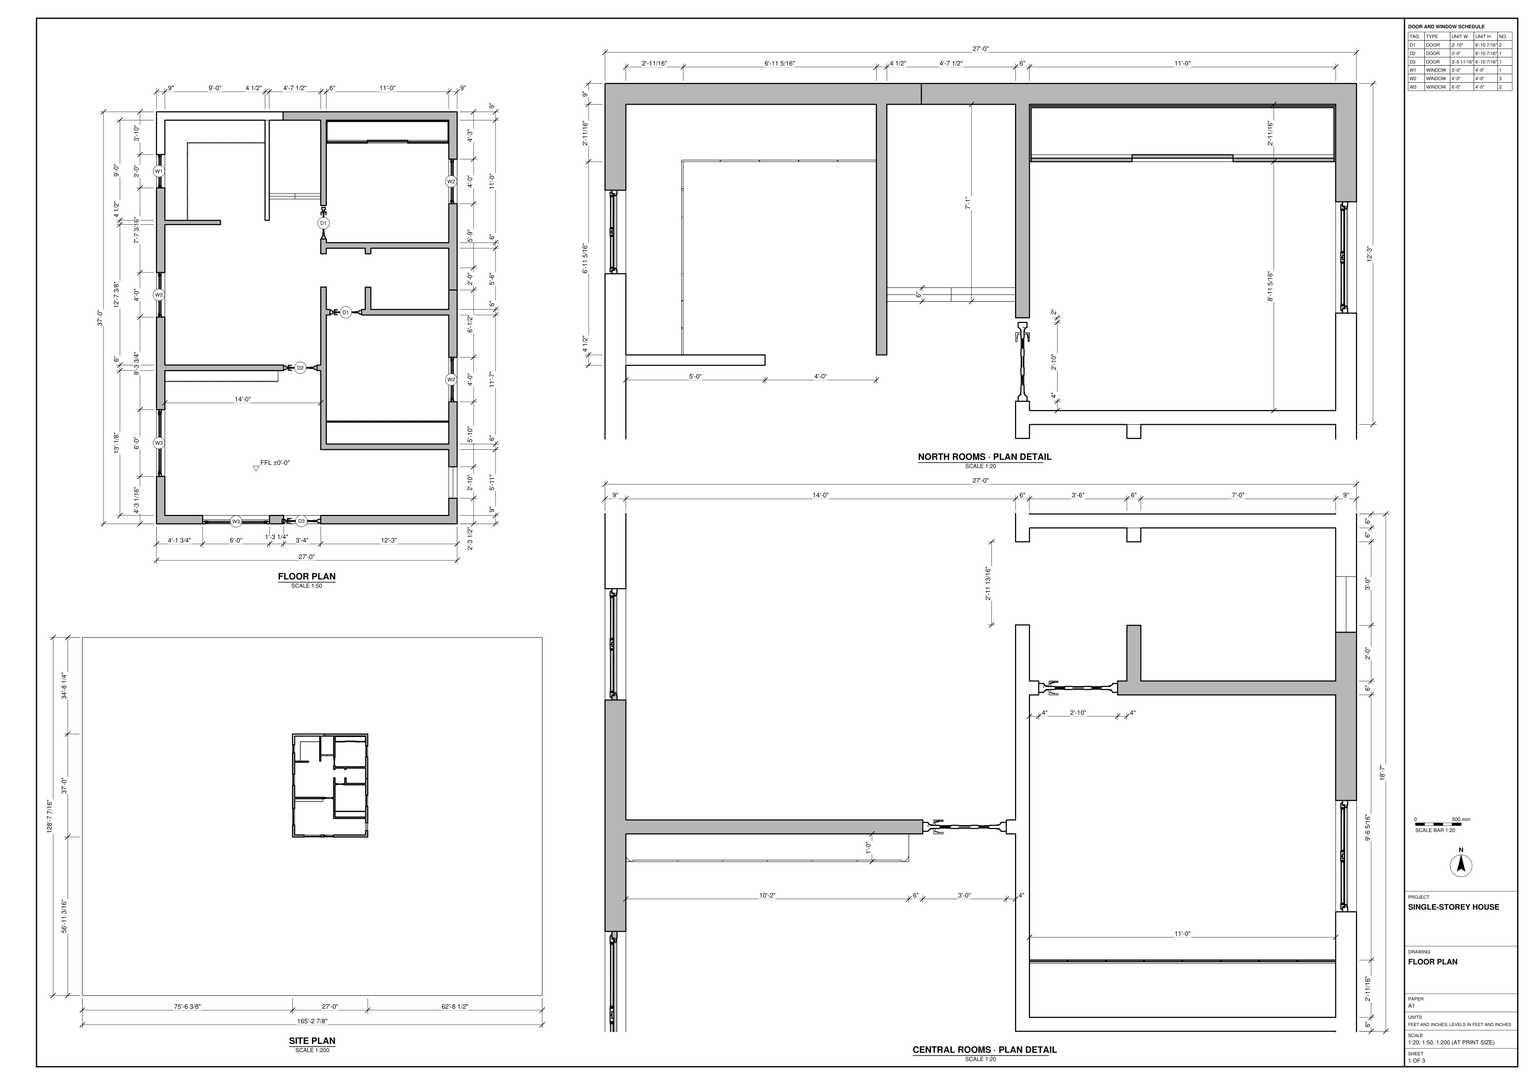
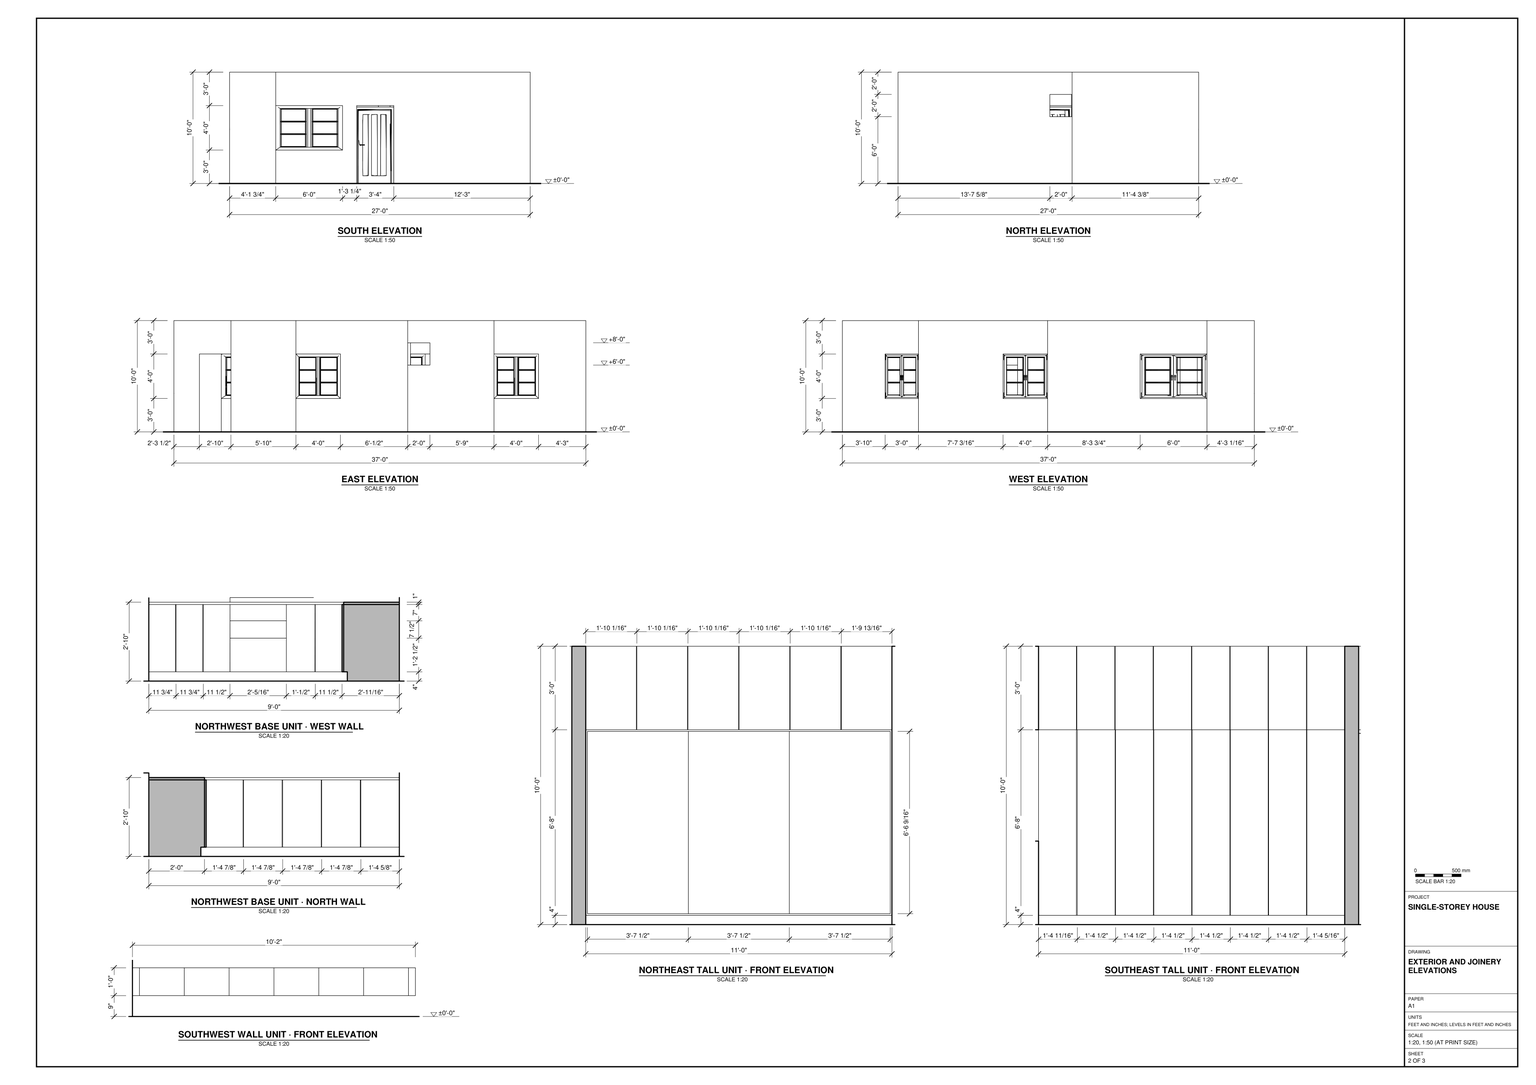
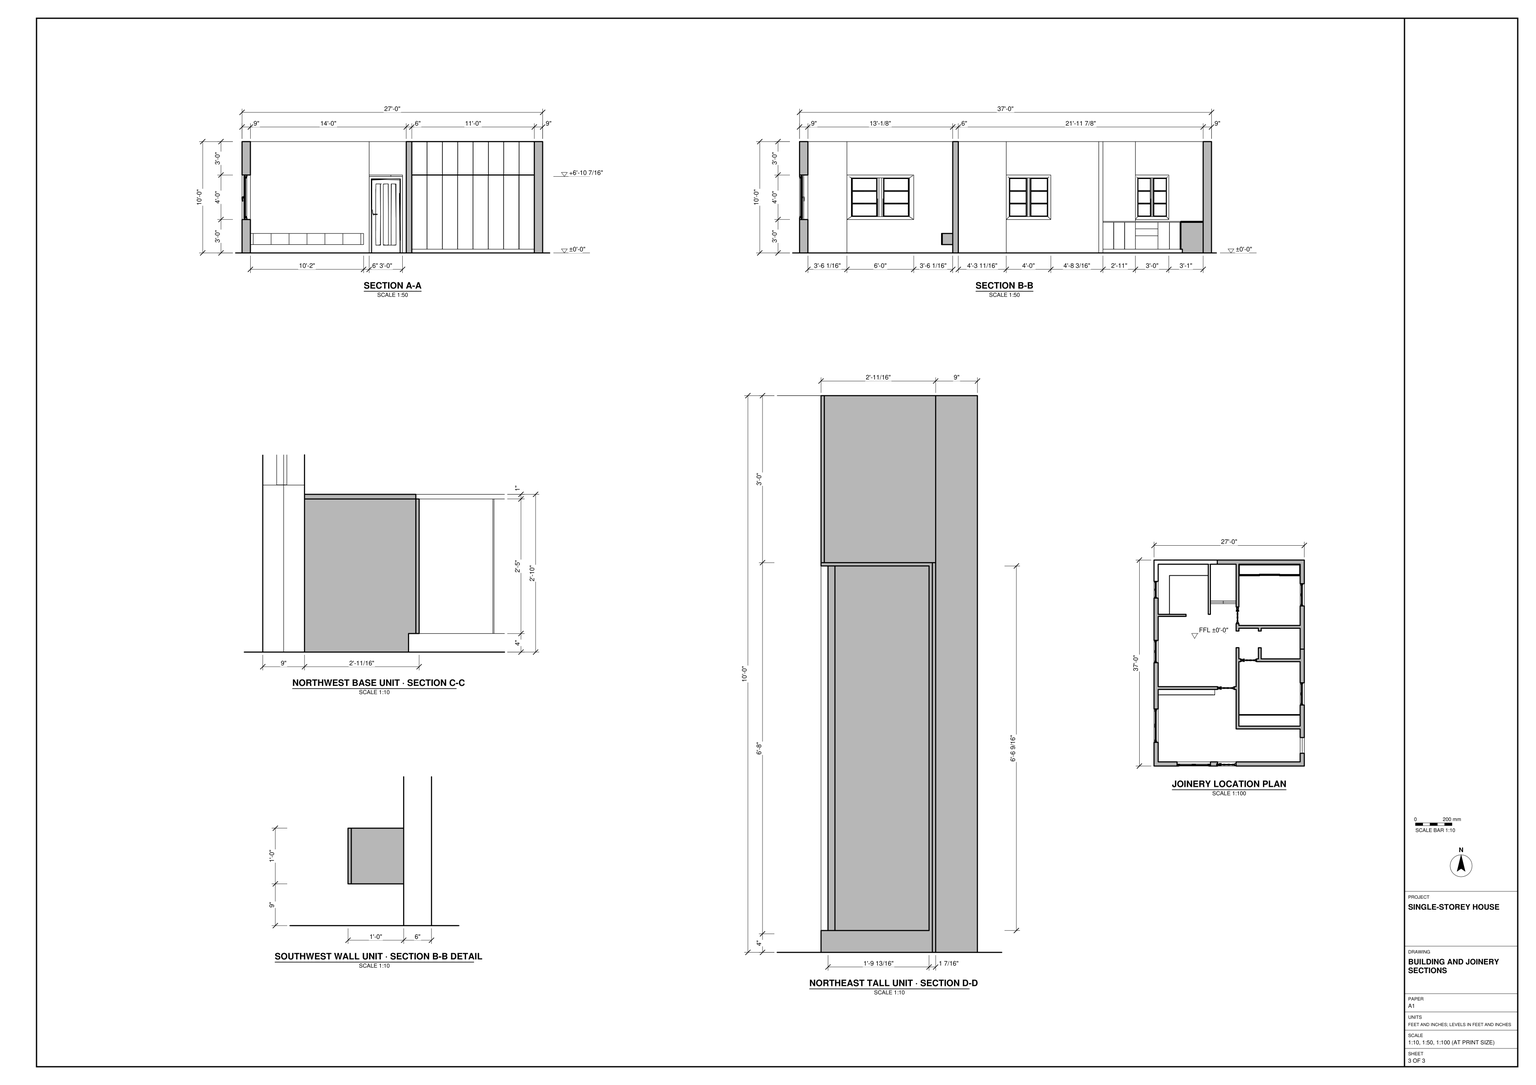
Build the house and its rectangular site in SketchUp from task_files/diagram_01.pdf. Work in feet and inches. The overall model measures 165'-2 7/8" east to west, 128'-7 7/16" north to south and 10'-0" high. The house footprint is 27'-0" east to west by 37'-0" north to south. Use the setbacks on the site plan to position it, with the entrance on the south side and the single finished floor at ±0'-0".

Model the floor, the 9" exterior walls and the interior partitions at their drawn thicknesses. Use the enlarged plans to locate the partition ends, doorways and passages between rooms. Fit the scheduled doors and windows, and use the elevations to set the sill heights and locate the smaller high openings on the north and east walls.

Build the base cabinetry around the northwest corner, the low wall-mounted unit in the southwest room and the full-height storage units in the northeast and southeast rooms. Follow the joinery elevations for the panel divisions and the sections for the cabinet depths, plinths and clearance above the floor. Keep shell elements and individual joinery pieces in separate groups or components, and use components for repeated parts. Decor and loose items, where shown, may be any suitable library component. Save one SketchUp model as output_files/single_storey_house_with_built_in_joinery_on_its_site.skp.

# SketchUp Ruby script. Lengths in inches.
U = 1.inch
M = Sketchup.active_model
def pt(a) = Geom::Point3d.new(a.map { |v| v * U })
def face(e, loops, mat)
  f = e.add_face(loops[0].map { |a| pt(a) })
  loops[1..].each { |l| e.add_face(l.map { |a| pt(a) }).erase! }
  f.material = f.back_material = mat if mat
  f
end
# faces: each face lists its corners as indices into pts; further lists are holes
def faces(e, pts, list, mat = nil) = list.each { |f| face(e, (f[0].is_a?(Array) ? f : [f]).map { |l| l.map { |i| pts[i] } }, mat) }
# xy, xz, yz: faces in a plane at the given z, y or x. An outline is a flat list of corners, or four numbers for a rectangle; further outlines are holes
def ring(l) = l.size == 4 ? [[l[0], l[1]], [l[2], l[1]], [l[2], l[3]], [l[0], l[3]]] : l.each_slice(2).to_a
def flat(e, list, mat, &to3) = list.each { |f| face(e, (f[0].is_a?(Array) ? f : [f]).map { |l| ring(l).map { |u, v| to3.(u, v) } }, mat) }
def xy(e, z, list, mat = nil) = flat(e, list, mat) { |x, y| [x, y, z] }
def xz(e, y, list, mat = nil) = flat(e, list, mat) { |x, z| [x, y, z] }
def yz(e, x, list, mat = nil) = flat(e, list, mat) { |y, z| [x, y, z] }
def lines(e, pts, list) = list.each { |a, b| e.add_line(pt(pts[a]), pt(pts[b])) }
# prism: a flat outline (further loops are holes) pulled along v
def prism(e, loops, v, mat = nil)
  f = face(e, loops, mat); d = Geom::Vector3d.new(v.map { |x| x * U })
  f.pushpull(f.normal.samedirection?(d) ? d.length : -d.length)
end
def box(e, o, s, mat = nil) = prism(e, [[o, [o[0] + s[0], o[1], o[2]], [o[0] + s[0], o[1] + s[1], o[2]], [o[0], o[1] + s[1], o[2]]]], [0, 0, s[2]], mat)
def at(x, y, z, deg = 0) = Geom::Transformation.translation(pt([x, y, z])) * Geom::Transformation.rotation(ORIGIN, Z_AXIS, deg.degrees)
def axes(o, x, y, z) = Geom::Transformation.new([*x, 0, *y, 0, *z, 0, *pt(o).to_a, 1])
def part(name) = M.definitions.add(name)
# library, detail: a bought-in or finely detailed component or shape, given as its bounding box
def library(name, o, s) = part(name).tap { |d| box(d.entities, o, s) }
def detail(e, o, s) = box(e.add_group.entities, o, s)
def put(e, d, t, mat = nil) = e.add_instance(d, t).tap { |i| i.material = mat if mat }
def group(e, t, mat = nil) = e.add_group.tap { |g| g.transformation = t; g.material = mat if mat }.entities
root = M.entities
M.materials.add("[Color B01]").color = [255, 216, 204]
M.materials.add("[Color L01]").color = [255, 204, 229]
M.materials.add("[Color M04]").color = [142, 142, 142]
M.materials.add("[Marble Carrara Gold Floor Tile]").color = [225, 223, 217]
M.materials.add("[Wood Cherry Original]").color = [152, 86, 42]
c1 = library("Window 46-30",[-29.96,-2.6,0],[59.92,5.19,59.84])
c2 = library("Door 243 067",[-20.85,-3,0],[41.7,6,82.46])
c3 = part("Group\#11")
box(c3.entities,[0,0,0],[43.53,1.5,78.58])
c4 = part("Group\#12")
box(c4.entities,[0.2,0,0],[21.8,0.71,36])
c5 = part("Group\#18")
prism(c5.entities,[[[0.71,0,0],[0.71,11.48,0],[0.71,11.52,29],[0.71,0,29]]],[-0.71,0,0])
c6 = part("Group\#15")
box(c6.entities,[0.2,0,0],[16.6,0.71,29])
c7 = part("Group\#24")
box(c7.entities,[0,0,0],[16.3,0.71,80])
c8 = part("Group\#23")
box(c8.entities,[0,0,0],[16.3,0.71,36])
c9 = part("Group\#25")
box(c9.entities,[0,0,0],[19.33,0.71,12])
xy(root,0,[[[0,0,1982.875,1543.4375],[906.4,683.1875,1230.4,1127.1875]],[956.14,683.1875,1028.14,687.6875],[1028.14,683.1875,1043.4,692.1875],[1043.4,683.1875,1083.4,692.1875],[1083.4,683.1875,1230.4,683.1875,1230.4,710.6875,1221.4,710.6875,1221.4,692.1875,1083.4,692.1875],
  [956.14,687.6875,1028.14,692.1875],[1221.4,710.6875,1225.9,744.6875],[1225.9,710.6875,1230.4,744.6875],[906.4,734.24,910.9,806.24],[910.9,734.24,915.4,806.24],
  [1221.4,744.6875,1230.4,744.6875,1230.4,814.6875,1221.4,814.6875,1221.4,769.1875,1089.4,769.1875,1089.4,908.1875,1093.4,908.1875,1093.4,914.1875,1089.4,914.1875,1089.4,938.35,1083.4,938.35,1083.4,854.3,1079.4,854.3,1079.4,848.3,1083.4,848.3,1083.4,763.1875,1221.4,763.1875],[1089.4,769.1875,1221.4,792.4],[1221.4,814.6875,1225.9,862.6875],[1225.9,814.6875,1230.4,862.6875],[915.4,836.3,1037.4,848.3],
  [906.4,905.99,910.9,953.99],[910.9,905.99,915.4,953.99],[1221.4,935.1875,1225.9,959.1875],[1225.9,935.1875,1230.4,959.1875],[906.4,953.99,915.4,1045.1875],
  [1131.4,974.1875,1137.4,980.1875],[915.4,1005.6875,975.4,1010.1875],[915.4,1010.1875,939.4,1010.1875,939.4,1094.1875,1023.4,1094.1875,1023.4,1118.1875,915.4,1118.1875],[1083.4,1026.1875,1089.4,1118.1875],[1221.4,1028.1875,1225.9,1076.1875],
  [1225.9,1028.1875,1230.4,1076.1875],[1027.9,1033.1875,1055.65,1036.1875],[1055.65,1033.1875,1083.4,1036.1875],[1027.9,1036.1875,1055.65,1039.1875],[1055.65,1036.1875,1083.4,1039.1875],
  [1027.9,1039.1875,1083.4,1118.1875],[906.4,1045.1875,910.9,1081.1875],[910.9,1045.1875,915.4,1081.1875],[1221.4,1076.1875,1230.4,1076.1875,1230.4,1127.1875,1066.8,1127.1875,1066.8,1118.1875,1221.4,1118.1875],[906.4,1081.1875,915.4,1081.1875,915.4,1118.1875,1042.8,1118.1875,1042.8,1127.1875,906.4,1127.1875],
  [1089.4,1094.1875,1221.4,1118.1875],[1042.8,1118.1875,1066.8,1122.6875],[1042.8,1122.6875,1066.8,1127.1875]])
xy(root,0,[[915.4,692.1875,1221.4,692.1875,1221.4,763.1875,1083.4,763.1875,1083.4,848.3,1079.4,848.3,1079.4,854.3,1083.4,854.3,1083.4,938.35,1089.4,938.35,1089.4,914.1875,1093.4,914.1875,1093.4,908.1875,1089.4,908.1875,1089.4,792.4,1221.4,792.4,1221.4,908.1875,1127.4,908.1875,1127.4,914.1875,1131.4,914.1875,1131.4,938.1875,1137.4,938.1875,1137.4,914.1875,1221.4,914.1875,1221.4,980.1875,1137.4,980.1875,1137.4,974.1875,1131.4,974.1875,1131.4,980.1875,1089.4,980.1875,1089.4,974.1875,1083.4,974.1875,1083.4,990.1875,1089.4,990.1875,1089.4,986.1875,1221.4,986.1875,1221.4,1094.1875,1089.4,1094.1875,1089.4,1026.1875,1083.4,1026.1875,1083.4,1033.1875,1027.9,1033.1875,1027.9,1118.1875,1023.4,1118.1875,1023.4,1094.1875,939.4,1094.1875,939.4,1010.1875,975.4,1010.1875,975.4,1005.6875,915.4,1005.6875,915.4,854.3,1043.4,854.3,1043.4,848.3,1037.4,848.3,1037.4,836.3,915.4,836.3]],"[Marble Carrara Gold Floor Tile]")
xy(root,4,[[1089.4,792.4,1221.4,793.1875]])
xy(root,84,[[1089.4,769.1875,1221.4,793.1875]])
xy(root,120,[[1089.4,769.1875,1221.4,793.1875]],"[Color L01]")
xz(root,769.1875,[[1089.4,0,1221.4,84],[1089.4,84,1221.4,120]])
xz(root,792.4,[[1089.4,0,1221.4,4]],"[Color L01]")
xz(root,793.1875,[[1089.4,4,1105.9,84],[1105.9,4,1122.4,84],[1122.4,4,1221.4,84],[1089.4,84,1221.4,120]])
yz(root,1089.4,[[769.1875,0,769.1875,84,793.1875,84,793.1875,4,792.4,4,792.4,0],[769.1875,84,793.1875,120]])
yz(root,1221.4,[[769.1875,0,792.4,0,792.4,4,793.1875,4,793.1875,84,769.1875,84],[769.1875,84,793.1875,120]])
p = [[1023.4,1094.1875,0],[1023.4,1010.1875,0]]
lines(root,p,[[0,1]])
put(root,c1,axes([1224,1052.1875,36],[0,-0.8011,0],[1,0,0],[0,0,0.80216]))
put(root,c1,axes([1224,838.6875,36],[0,-0.8011,0],[1,0,0],[0,0,0.80216]))
put(root,c1,axes([909,929.99,36],[0,-0.8011,0],[1,0,0],[0,0,0.80216]))
put(root,c1,axes([909,1063.1875,36],[0,-0.60083,0],[1,0,0],[0,0,0.80216]))
put(root,c1,axes([909,770.24,36],[0,-1.20165,0],[1,0,0],[0,0,0.80216]))
put(root,c1,axes([992.14,685.78,36],[-1.20165,0,0],[0,-1,0],[0,0,0.80216]))
put(root,c2,at(1062.55,686.1875,0))
put(root,c2,axes([1061.4,851.3,0],[0.86337,0,0],[0,1,0],[0,0,1]))
put(root,c2,axes([1110.4,911.1875,0],[0.8154,0,0],[0,1,0],[0,0,1]))
put(root,c2,axes([1086.4,1007.1875,0],[0,-0.8154,0],[1,0,0],[0,0,1]))
g1 = group(root,at(1079.4,744.6875,0))
xy(g1,0,[[142,0,142,18.5,4,18.5,4,103.61,0,103.61,0,109.61,4,109.61,4,193.67,10,193.67,10,169.5,14,169.5,14,163.5,10,163.5,10,24.5,142,24.5,142,70,151,70,151,0]])
xy(g1,84,[[-36,103.61,0,109.61]])
xy(g1,120,[[142,0,151,0,151,70,142,70,142,24.5,10,24.5,10,163.5,14,163.5,14,169.5,10,169.5,10,193.67,4,193.67,4,109.61,-36,109.61,-36,103.61,4,103.61,4,18.5,142,18.5]])
xz(g1,0,[[142,0,146.5,120],[146.5,0,151,120]])
xz(g1,18.5,[[4,0,142,120]])
xz(g1,24.5,[[10,0,142,120]])
xz(g1,70,[[142,0,146.5,120],[146.5,0,151,120]])
xz(g1,103.61,[[0,0,4,0,4,120,-36,120,-36,84,0,84]])
xz(g1,109.61,[[0,0,0,84,-36,84,-36,120,4,120,4,0]])
xz(g1,163.5,[[10,0,14,120]])
xz(g1,169.5,[[10,0,14,120]])
xz(g1,193.67,[[4,0,10,120]])
yz(g1,-36,[[103.61,84,109.61,120]])
yz(g1,0,[[103.61,0,109.61,84]])
yz(g1,4,[[18.5,0,103.61,120],[109.61,0,193.67,120]])
yz(g1,10,[[24.5,0,163.5,120],[169.5,0,193.67,120]])
yz(g1,14,[[163.5,0,169.5,120]])
yz(g1,142,[[0,0,18.5,120],[24.5,0,70,120]])
yz(g1,151,[[0,0,70,120]])
g2 = group(root,at(906.4,683.1875,0))
prism(g2,[[[9,51.06,0],[9,9,0],[49.74,9,0],[49.74,4.5,0],[49.74,0,0],[0,0,0],[0,51.06,0],[4.5,51.06,0]]],[0,0,120])
g3 = group(root,at(906.4,806.24,0))
xy(g3,0,[[0,-72,0,99.75,9,99.75,9,48.06,137,48.06,137,42.06,9,42.06,9,-72]])
xy(g3,36,[[0,-72,9,0]])
xy(g3,84,[[0,-72,9,0]])
xy(g3,120,[[0,-72,9,-72,9,42.06,137,42.06,137,48.06,9,48.06,9,99.75,0,99.75]])
xz(g3,-72,[[0,0,9,36],[0,84,9,120]])
xz(g3,0,[[0,36,9,84]])
xz(g3,42.06,[[9,0,137,120]])
xz(g3,48.06,[[9,0,137,120]])
xz(g3,99.75,[[0,0,4.5,120],[4.5,0,9,120]])
yz(g3,0,[[-72,0,-72,36,0,36,0,84,-72,84,-72,120,99.75,120,99.75,0]])
yz(g3,9,[[-72,0,42.06,0,42.06,120,-72,120,-72,84,0,84,0,36,-72,36],[48.06,0,99.75,120]])
yz(g3,137,[[42.06,0,48.06,120]])
g4 = group(root,at(906.4,953.99,0))
xy(g4,0,[[0,-48,0,91.2,9,91.2,9,56.19,69,56.19,69,51.69,9,51.69,9,-48]])
xy(g4,36,[[0,-48,9,0]])
xy(g4,84,[[0,-48,9,0]])
xy(g4,120,[[0,-48,9,-48,9,51.69,69,51.69,69,56.19,9,56.19,9,91.2,0,91.2]])
xz(g4,-48,[[0,0,9,36],[0,84,9,120]])
xz(g4,0,[[0,36,9,84]])
xz(g4,51.69,[[9,0,69,120]])
xz(g4,56.19,[[9,0,69,120]])
xz(g4,91.2,[[0,0,4.5,120],[4.5,0,9,120]])
yz(g4,0,[[-48,0,-48,36,0,36,0,84,-48,84,-48,120,91.2,120,91.2,0]])
yz(g4,9,[[-48,0,51.69,0,51.69,120,-48,120,-48,84,0,84,0,36,-48,36],[56.19,0,91.2,120]])
yz(g4,69,[[51.69,0,56.19,120]])
g5 = group(root,at(906.4,1081.1875,0))
xy(g5,0,[[117,-71,117,37,9,37,9,-36,0,-36,0,46,136.4,46,136.4,37,121.5,37,121.5,-71]])
xy(g5,36,[[0,-36,4.5,0],[4.5,-36,9,0]])
xy(g5,84,[[0,-36,4.5,0],[4.5,-36,9,0]])
xy(g5,120,[[117,-71,121.5,-71,121.5,37,136.4,37,136.4,46,0,46,0,-36,9,-36,9,37,117,37]])
xz(g5,-71,[[117,0,121.5,120]])
xz(g5,-36,[[0,0,9,36],[0,84,9,120]])
xz(g5,0,[[0,36,4.5,84],[4.5,36,9,84]])
xz(g5,37,[[9,0,117,120],[121.5,0,136.4,120]])
xz(g5,46,[[0,0,136.4,120]])
yz(g5,0,[[-36,0,-36,36,0,36,0,84,-36,84,-36,120,46,120,46,0]])
yz(g5,9,[[-36,0,37,0,37,120,-36,120,-36,84,0,84,0,36,-36,36]])
yz(g5,117,[[-71,0,37,120]])
yz(g5,121.5,[[-71,0,37,120]])
yz(g5,136.4,[[37,0,41.5,120],[41.5,0,46,120]])
g6 = group(root,at(1066.8,1076.1875,0))
xy(g6,0,[[16.6,-50,16.6,42,-24,42,-24,51,163.6,51,163.6,-48,154.6,-48,154.6,42,22.6,42,22.6,-50]])
xy(g6,36,[[154.6,-48,159.1,0],[159.1,-48,163.6,0]])
xy(g6,72,[[-24,42,0,51]])
xy(g6,84,[[154.6,-48,159.1,0],[159.1,-48,163.6,0]])
xy(g6,96,[[-24,42,0,51]])
xy(g6,120,[[16.6,-50,22.6,-50,22.6,42,154.6,42,154.6,-48,163.6,-48,163.6,51,-24,51,-24,42,16.6,42]])
xz(g6,-50,[[16.6,0,22.6,120]])
xz(g6,-48,[[154.6,0,163.6,36],[154.6,84,163.6,120]])
xz(g6,0,[[154.6,36,159.1,84],[159.1,36,163.6,84]])
xz(g6,42,[[-24,0,16.6,0,16.6,120,-24,120,-24,96,0,96,0,72,-24,72],[22.6,0,154.6,120]])
xz(g6,51,[[-24,0,-24,72,0,72,0,96,-24,96,-24,120,163.6,120,163.6,0]])
yz(g6,-24,[[42,0,51,72],[42,96,51,120]])
yz(g6,0,[[42,72,51,96]])
yz(g6,16.6,[[-50,0,42,120]])
yz(g6,22.6,[[-50,0,42,120]])
yz(g6,154.6,[[-48,0,-48,36,0,36,0,84,-48,84,-48,120,42,120,42,0]])
yz(g6,163.6,[[-48,0,51,0,51,120,-48,120,-48,84,0,84,0,36,-48,36]])
g7 = group(root,at(1083.4,959.1875,0))
xy(g7,0,[[138,-24,138,21,54,21,54,15,48,15,48,21,6,21,6,15,0,15,0,31,6,31,6,27,138,27,138,69,147,69,147,-24]])
xy(g7,72,[[138,-24,142.5,0],[142.5,-24,147,0]])
xy(g7,84,[[48,-21,54,15],[0,-20.83,6,15]])
xy(g7,96,[[138,-24,142.5,0],[142.5,-24,147,0]])
xy(g7,120,[[138,-24,147,-24,147,69,138,69,138,27,6,27,6,31,0,31,0,-20.83,6,-20.83,6,21,48,21,48,-21,54,-21,54,21,138,21]])
xz(g7,-24,[[138,0,147,72],[138,96,147,120]])
xz(g7,-21,[[48,84,54,120]])
xz(g7,-20.83,[[0,84,6,120]])
xz(g7,0,[[138,72,142.5,96],[142.5,72,147,96]])
xz(g7,15,[[0,0,6,84],[48,0,54,84]])
xz(g7,21,[[6,0,48,120],[54,0,138,120]])
xz(g7,27,[[6,0,138,120]])
xz(g7,31,[[0,0,6,120]])
xz(g7,69,[[138,0,142.5,120],[142.5,0,147,120]])
yz(g7,0,[[15,0,15,84,-20.83,84,-20.83,120,31,120,31,0]])
yz(g7,6,[[15,0,21,0,21,120,-20.83,120,-20.83,84,15,84],[27,0,31,120]])
yz(g7,48,[[15,0,15,84,-21,84,-21,120,21,120,21,0]])
yz(g7,54,[[15,0,21,0,21,120,-21,120,-21,84,15,84]])
yz(g7,138,[[-24,0,-24,72,0,72,0,96,-24,96,-24,120,21,120,21,0],[27,0,69,120]])
yz(g7,147,[[-24,0,69,0,69,120,-24,120,-24,96,0,96,0,72,-24,72]])
g8 = group(root,at(1127.4,862.6875,0))
xy(g8,0,[[94,-48,94,45.5,0,45.5,0,51.5,4,51.5,4,75.5,10,75.5,10,51.5,94,51.5,94,72.5,103,72.5,103,-48]])
xy(g8,36,[[94,-48,98.5,0],[98.5,-48,103,0]])
xy(g8,84,[[94,-48,98.5,0],[98.5,-48,103,0],[-34,45.5,0,51.5]])
xy(g8,120,[[94,-48,103,-48,103,72.5,94,72.5,94,51.5,10,51.5,10,75.5,4,75.5,4,51.5,-34,51.5,-34,45.5,94,45.5]])
xz(g8,-48,[[94,0,103,36],[94,84,103,120]])
xz(g8,0,[[94,36,98.5,84],[98.5,36,103,84]])
xz(g8,45.5,[[0,0,94,0,94,120,-34,120,-34,84,0,84]])
xz(g8,51.5,[[0,0,0,84,-34,84,-34,120,4,120,4,0],[10,0,94,120]])
xz(g8,72.5,[[94,0,98.5,120],[98.5,0,103,120]])
xz(g8,75.5,[[4,0,10,120]])
yz(g8,-34,[[45.5,84,51.5,120]])
yz(g8,0,[[45.5,0,51.5,84]])
yz(g8,4,[[51.5,0,75.5,120]])
yz(g8,10,[[51.5,0,75.5,120]])
yz(g8,94,[[-48,0,-48,36,0,36,0,84,-48,84,-48,120,45.5,120,45.5,0],[51.5,0,72.5,120]])
yz(g8,103,[[-48,0,72.5,0,72.5,120,-48,120,-48,84,0,84,0,36,-48,36]])
g9 = group(root,at(1028.14,683.1875,0))
xy(g9,0,[[-72,0,15.26,9],[55.26,0,55.26,9,193.26,9,193.26,27.5,202.26,27.5,202.26,0]])
xy(g9,36,[[-72,0,0,4.5],[-72,4.5,0,9]])
xy(g9,84,[[-72,0,0,4.5],[15.26,0,55.26,9],[-72,4.5,0,9],[193.26,27.5,197.76,61.5],[197.76,27.5,202.26,61.5]])
xy(g9,120,[[-72,0,202.26,0,202.26,61.5,193.26,61.5,193.26,9,-72,9]])
xz(g9,0,[[-72,0,15.26,0,15.26,84,55.26,84,55.26,0,202.26,0,202.26,120,-72,120,-72,84,0,84,0,36,-72,36]])
xz(g9,9,[[-72,0,-72,36,0,36,0,84,-72,84,-72,120,193.26,120,193.26,0,55.26,0,55.26,84,15.26,84,15.26,0]])
xz(g9,27.5,[[193.26,0,197.76,84],[197.76,0,202.26,84]])
xz(g9,61.5,[[193.26,84,202.26,120]])
yz(g9,-72,[[0,0,9,36],[0,84,9,120]])
yz(g9,0,[[0,36,4.5,84],[4.5,36,9,84]])
yz(g9,15.26,[[0,0,9,84]])
yz(g9,55.26,[[0,0,9,84]])
yz(g9,193.26,[[9,0,9,120,61.5,120,61.5,84,27.5,84,27.5,0]])
yz(g9,202.26,[[0,0,27.5,0,27.5,84,61.5,84,61.5,120,0,120]])
p = [[55.26,0,0],[15.26,0,0]]
lines(g9,p,[[0,1]])
g10 = group(root,at(1089.4,1093.48,0),"[Color B01]")
xy(g10,0,[[0,0,132,24]])
xy(g10,4.71,[[0.71,0,44.24,1.5],[44.24,0,87.76,1.5],[87.76,0,131.29,1.5],[0.71,1.5,44.24,3],[44.24,1.5,87.76,3],
  [87.76,1.5,131.29,3],[0.71,3,131.29,23.29]])
xy(g10,83.29,[[0.71,0,26.4,23.29],[26.4,0,52.8,23.29],[52.8,0,79.2,23.29],[79.2,0,105.6,23.29],[105.6,0,131.29,23.29]])
xy(g10,84,[[0,0,132,24]])
xz(g10,0,[[0,0,132,4],[[0,4,132,84],[0.71,4.71,131.29,83.29]]])
xz(g10,23.29,[[0.71,4.71,131.29,83.29]])
xz(g10,24,[[0,0,132,84]])
yz(g10,0,[[0,0,24,84]])
yz(g10,0.71,[[0,4.71,23.29,83.29]])
yz(g10,131.29,[[0,4.71,23.29,83.29]])
yz(g10,132,[[0,0,24,84]])
put(g10,c3,at(0.71,0,4.71))
g11 = group(g10,at(0,0.71,84))
put(g11,c4,at(110,-0.71,0))
g12 = group(g11,at(0,0,0))
xy(g12,0,[[0,0,132,24]])
xy(g12,36,[[0,0,132,24]])
xz(g12,0,[[0,0,110,36],[110,0,132,36]])
xz(g12,24,[[0,0,132,36]])
yz(g12,0,[[0,0,24,36]])
yz(g12,132,[[0,0,24,36]])
put(g11,c4,at(87.96,-0.71,0))
put(g11,c4,at(65.92,-0.71,0))
put(g11,c4,at(43.88,-0.71,0))
put(g11,c4,at(21.84,-0.71,0))
put(g11,c4,at(-0.2,-0.71,0))
put(g10,c3,at(87.76,0,4.71))
put(g10,c3,at(44.24,1.5,4.71))
g13 = group(root,at(915.4,1010.1875,0),"[Color M04]")
xy(g13,0,[[0,0,0,108,108,108,108,85.57,22.43,85.57,22.43,0]])
xy(g13,4,[[22.43,0,24,84],[22.43,84,108,85.57]])
xy(g13,33,[[0,0,24,0,24,84,108,84,108,108,0,108]])
xz(g13,0,[[0,0,22.43,0,22.43,4,24,4,24,33,0,33]])
xz(g13,84,[[24,4,91.2,33],[91.2,4,108,33]])
xz(g13,85.57,[[22.43,0,108,4]])
xz(g13,108,[[0,0,108,33]])
yz(g13,0,[[0,0,35,33],[35,0,71,33],[71,0,108,33]])
yz(g13,22.43,[[0,0,85.57,4]])
yz(g13,24,[[0,4,11.48,4,11.52,33,0,33],[11.48,4,23.01,4,23.05,33,11.52,33],[23.01,4,35.01,4,35.01,33,23.05,33],[35.01,4,59.29,18.5],[59.29,4,71.65,33],
  [71.65,4,84,33],[35.01,18.5,59.29,25.94],[35.01,25.94,59.29,33]])
yz(g13,108,[[85.57,0,108,0,108,33,84,33,84,4,85.57,4]])
g14 = group(g13,at(24,35.01,4))
box(g14,[0,0,0],[0.71,24.29,14.5])
put(g13,c5,at(24,0,4))
g15 = group(g13,at(24,59.29,4))
prism(g15,[[[0.71,0,0],[0.71,11.48,0],[0.71,12.3125,0],[0.71,12.35,29],[0.71,11.52,29],[0.71,0,29]]],[-0.71,0,0])
g16 = group(g13,at(24,35.01,18.5))
box(g16,[0,0,0],[0.71,24.29,7.5])
g17 = group(g13,at(24,35.01,26))
box(g17,[0,0,0],[0.71,24.29,7])
put(g13,c5,at(24,71.77,4))
put(g13,c5,at(24,11.74,4))
put(g13,c5,at(24,23.48,4))
put(g13,c6,at(57.5,83.29,4))
put(g13,c6,at(40.65,83.29,4))
put(g13,c6,at(23.8,83.29,4))
put(g13,c6,at(91.2,83.29,4))
put(g13,c6,at(74.35,83.29,4))
g18 = group(g13,at(0,0,33))
prism(g18,[[[24,84,0],[24,0,0],[0,0,0],[0,35,0],[0,71,0],[0,108,0],[108,108,0],[108,84,0]]],[0,0,1])
put(root,c7,at(1089.4,793.1875,4),"[Color L01]")
put(root,c7,at(1105.9,793.1875,4),"[Color L01]")
put(root,c7,at(1122.4,793.1875,4),"[Color L01]")
put(root,c7,at(1138.9,793.1875,4),"[Color L01]")
put(root,c7,at(1155.4,793.1875,4),"[Color L01]")
put(root,c7,at(1171.9,793.1875,4),"[Color L01]")
put(root,c7,at(1188.4,793.1875,4),"[Color L01]")
put(root,c7,at(1205.1,793.1875,4),"[Color L01]")
put(root,c8,at(1205.1,793.1875,84),"[Color L01]")
put(root,c8,at(1188.57,793.1875,84),"[Color L01]")
put(root,c8,at(1172.04,793.1875,84),"[Color L01]")
put(root,c8,at(1155.51,793.1875,84),"[Color L01]")
put(root,c8,at(1138.98,793.1875,84),"[Color L01]")
put(root,c8,at(1122.46,793.1875,84),"[Color L01]")
put(root,c8,at(1105.93,793.1875,84),"[Color L01]")
put(root,c8,at(1089.4,793.1875,84),"[Color L01]")
g19 = group(root,at(915.4,836.3,9))
xy(g19,0,[[3.01,0,2.62,0.03,2.23,0.1,1.86,0.23,1.51,0.4,1.18,0.62,0.89,0.88,0.625,1.17,0.41,1.5,0.23,1.85,0.1,2.22,0.03,2.61,0,3,0,12,122,12,122,3,121.97,2.61,121.9,2.22,121.77,1.85,121.6,1.5,121.38,1.17,121.12,0.88,120.83,0.62,120.5,0.4,120.15,0.23,119.78,0.1,119.39,0.03,119,0,119,0.71,3.01,0.71]])
xy(g19,12,[[3.01,0,3.01,0.71,119,0.71,119,0,119.39,0.03,119.78,0.1,120.15,0.23,120.5,0.4,120.83,0.62,121.12,0.88,121.38,1.17,121.6,1.5,121.77,1.85,121.9,2.22,121.97,2.61,122,3,122,12,0,12,0,3,0.03,2.61,0.1,2.22,0.23,1.85,0.41,1.5,0.625,1.17,0.89,0.88,1.18,0.62,1.51,0.4,1.86,0.23,2.23,0.1,2.62,0.03]],"[Wood Cherry Original]")
xz(g19,0.71,[[3.01,0,80.34,12],[80.34,0,99.67,12],[99.67,0,119,12]])
xz(g19,12,[[0,0,122,12]],"[Wood Cherry Original]")
yz(g19,0,[[3,0,12,12]],"[Wood Cherry Original]")
yz(g19,3.01,[[0,0,0.71,12]])
yz(g19,119,[[0,0,0.71,12]])
yz(g19,122,[[3,0,12,12]],"[Wood Cherry Original]")
p = [[2.62,0.03,12],[2.23,0.1,12],[2.23,0.1,0],[2.62,0.03,0],[3.01,0,12],[3.01,0,0],
  [119.39,0.03,12],[119,0,12],[119,0,0],[119.39,0.03,0],[119.78,0.1,12],[119.78,0.1,0],
  [1.86,0.23,12],[1.86,0.23,0],[120.15,0.23,12],[120.15,0.23,0],[1.51,0.4,12],[1.51,0.4,0],
  [120.5,0.4,12],[120.5,0.4,0],[1.18,0.62,12],[1.18,0.62,0],[120.83,0.62,12],[120.83,0.62,0],
  [0.89,0.88,12],[0.89,0.88,0],[121.12,0.88,12],[121.12,0.88,0],[0.625,1.17,12],[0.625,1.17,0],
  [121.38,1.17,12],[121.38,1.17,0],[0.41,1.5,12],[0.41,1.5,0],[121.6,1.5,12],[121.6,1.5,0],
  [0.23,1.85,12],[0.23,1.85,0],[121.77,1.85,12],[121.77,1.85,0],[0.1,2.22,12],[0.1,2.22,0],
  [121.9,2.22,12],[121.9,2.22,0],[0.03,2.61,12],[0.03,2.61,0],[121.97,2.61,12],[121.97,2.61,0],
  [0,3,12],[0,3,0],[122,3,12],[122,3,0]]
faces(g19,p,[[0,1,2,3],[4,0,3,5],[6,7,8,9],[10,6,9,11],[1,12,13,2],[14,10,11,15],[12,16,17,13],[18,14,15,19],
  [16,20,21,17],[22,18,19,23],[20,24,25,21],[26,22,23,27],[24,28,29,25],[30,26,27,31],[28,32,33,29],[34,30,31,35],
  [32,36,37,33],[38,34,35,39],[36,40,41,37],[42,38,39,43],[40,44,45,41],[46,42,43,47],[44,48,49,45],[50,46,47,51]],"[Wood Cherry Original]")
put(g19,c9,at(80.34,0,0),"[Wood Cherry Original]")
put(g19,c9,at(22.34,0,0),"[Wood Cherry Original]")
put(g19,c9,at(61.01,0,0),"[Wood Cherry Original]")
put(g19,c9,at(41.67,0,0),"[Wood Cherry Original]")
put(g19,c9,at(99.67,0,0),"[Wood Cherry Original]")
put(g19,c9,at(3.01,0,0),"[Wood Cherry Original]")
